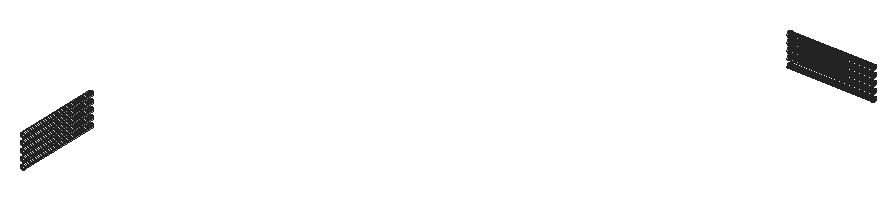
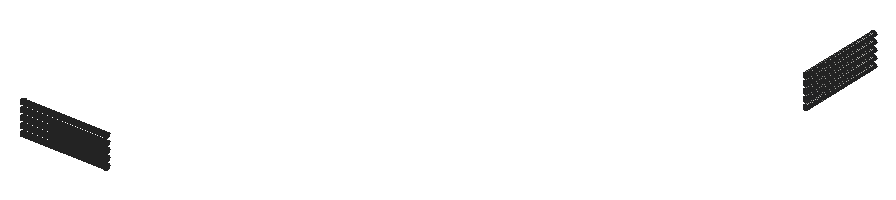
# SketchUp Ruby script. Lengths in inches.
U = 1.inch
M = Sketchup.active_model
def pt(a) = Geom::Point3d.new(a.map { |v| v * U })
def face(e, loops, mat)
  f = e.add_face(loops[0].map { |a| pt(a) })
  loops[1..].each { |l| e.add_face(l.map { |a| pt(a) }).erase! }
  f.material = f.back_material = mat if mat
  f
end
# faces: each face lists its corners as indices into pts; further lists are holes
def faces(e, pts, list, mat = nil) = list.each { |f| face(e, (f[0].is_a?(Array) ? f : [f]).map { |l| l.map { |i| pts[i] } }, mat) }
# xy, xz, yz: faces in a plane at the given z, y or x. An outline is a flat list of corners, or four numbers for a rectangle; further outlines are holes
def ring(l) = l.size == 4 ? [[l[0], l[1]], [l[2], l[1]], [l[2], l[3]], [l[0], l[3]]] : l.each_slice(2).to_a
def flat(e, list, mat, &to3) = list.each { |f| face(e, (f[0].is_a?(Array) ? f : [f]).map { |l| ring(l).map { |u, v| to3.(u, v) } }, mat) }
def xy(e, z, list, mat = nil) = flat(e, list, mat) { |x, y| [x, y, z] }
def xz(e, y, list, mat = nil) = flat(e, list, mat) { |x, z| [x, y, z] }
def yz(e, x, list, mat = nil) = flat(e, list, mat) { |y, z| [x, y, z] }
def lines(e, pts, list) = list.each { |a, b| e.add_line(pt(pts[a]), pt(pts[b])) }
# prism: a flat outline (further loops are holes) pulled along v
def prism(e, loops, v, mat = nil)
  f = face(e, loops, mat); d = Geom::Vector3d.new(v.map { |x| x * U })
  f.pushpull(f.normal.samedirection?(d) ? d.length : -d.length)
end
def box(e, o, s, mat = nil) = prism(e, [[o, [o[0] + s[0], o[1], o[2]], [o[0] + s[0], o[1] + s[1], o[2]], [o[0], o[1] + s[1], o[2]]]], [0, 0, s[2]], mat)
def at(x, y, z, deg = 0) = Geom::Transformation.translation(pt([x, y, z])) * Geom::Transformation.rotation(ORIGIN, Z_AXIS, deg.degrees)
def axes(o, x, y, z) = Geom::Transformation.new([*x, 0, *y, 0, *z, 0, *pt(o).to_a, 1])
def part(name) = M.definitions.add(name)
# library, detail: a bought-in or finely detailed component or shape, given as its bounding box
def library(name, o, s) = part(name).tap { |d| box(d.entities, o, s) }
def detail(e, o, s) = box(e.add_group.entities, o, s)
def put(e, d, t, mat = nil) = e.add_instance(d, t).tap { |i| i.material = mat if mat }
def group(e, t, mat = nil) = e.add_group.tap { |g| g.transformation = t; g.material = mat if mat }.entities
root = M.entities
p = [[83.53,662.8,1317.02],[82.57,662.8,1317.14],[82.57,806.17,1317.14],[83.53,806.17,1317.02],[84.48,662.8,1317.14],[84.48,806.17,1317.14],
  [697.99,1500.33,1317.14],[697.99,1501.28,1317.02],[841.36,1501.28,1317.02],[841.36,1500.33,1317.14],[697.99,1502.24,1317.14],[841.36,1502.24,1317.14],
  [81.68,662.8,1317.51],[81.68,806.17,1317.51],[85.37,662.8,1317.51],[85.37,806.17,1317.51],[697.99,1499.44,1317.51],[841.36,1499.44,1317.51],
  [697.99,1503.13,1317.51],[841.36,1503.13,1317.51],[80.92,662.8,1318.1],[80.92,806.17,1318.1],[86.13,662.8,1318.1],[86.13,806.17,1318.1],
  [697.99,1498.68,1318.1],[841.36,1498.68,1318.1],[697.99,1503.89,1318.1],[841.36,1503.89,1318.1],[80.33,662.8,1318.86],[80.33,806.17,1318.86],
  [86.72,662.8,1318.86],[86.72,806.17,1318.86],[697.99,1498.09,1318.86],[841.36,1498.09,1318.86],[697.99,1504.48,1318.86],[841.36,1504.48,1318.86],
  [79.97,662.8,1319.75],[79.97,806.17,1319.75],[87.09,662.8,1319.75],[87.09,806.17,1319.75],[697.99,1497.72,1319.75],[841.36,1497.72,1319.75],
  [697.99,1504.85,1319.75],[841.36,1504.85,1319.75],[79.84,662.8,1320.7],[79.84,806.17,1320.7],[87.21,662.8,1320.7],[87.21,806.17,1320.7],
  [697.99,1497.6,1320.7],[841.36,1497.6,1320.7],[697.99,1504.97,1320.7],[841.36,1504.97,1320.7],[79.97,662.8,1321.66],[79.97,806.17,1321.66],
  [87.09,662.8,1321.66],[87.09,806.17,1321.66],[697.99,1497.72,1321.66],[841.36,1497.72,1321.66],[697.99,1504.85,1321.66],[841.36,1504.85,1321.66],
  [80.33,662.8,1322.55],[80.33,806.17,1322.55],[86.72,662.8,1322.55],[86.72,806.17,1322.55],[697.99,1498.09,1322.55],[841.36,1498.09,1322.55],
  [697.99,1504.48,1322.55],[841.36,1504.48,1322.55],[80.92,662.8,1323.3125],[80.92,806.17,1323.3125],[86.13,662.8,1323.3125],[86.13,806.17,1323.3125],
  [697.99,1498.68,1323.3125],[841.36,1498.68,1323.3125],[697.99,1503.89,1323.3125],[841.36,1503.89,1323.3125],[81.68,662.8,1323.9],[81.68,806.17,1323.9],
  [85.37,662.8,1323.9],[85.37,806.17,1323.9],[697.99,1499.44,1323.9],[841.36,1499.44,1323.9],[697.99,1503.13,1323.9],[841.36,1503.13,1323.9],
  [82.57,662.8,1324.27],[82.57,806.17,1324.27],[84.48,662.8,1324.27],[84.48,806.17,1324.27],[697.99,1500.33,1324.27],[841.36,1500.33,1324.27],
  [697.99,1502.24,1324.27],[841.36,1502.24,1324.27],[83.53,662.8,1324.39],[83.53,806.17,1324.39],[697.99,1501.28,1324.39],[841.36,1501.28,1324.39],
  [83.53,662.8,1329.02],[82.57,662.8,1329.14],[82.57,806.17,1329.14],[83.53,806.17,1329.02],[84.48,662.8,1329.14],[84.48,806.17,1329.14],
  [697.99,1500.33,1329.14],[697.99,1501.28,1329.02],[841.36,1501.28,1329.02],[841.36,1500.33,1329.14],[697.99,1502.24,1329.14],[841.36,1502.24,1329.14],
  [81.68,662.8,1329.51],[81.68,806.17,1329.51],[85.37,662.8,1329.51],[85.37,806.17,1329.51],[697.99,1499.44,1329.51],[841.36,1499.44,1329.51],
  [697.99,1503.13,1329.51],[841.36,1503.13,1329.51],[80.92,662.8,1330.1],[80.92,806.17,1330.1],[86.13,662.8,1330.1],[86.13,806.17,1330.1],
  [697.99,1498.68,1330.1],[841.36,1498.68,1330.1],[697.99,1503.89,1330.1],[841.36,1503.89,1330.1],[80.33,662.8,1330.86],[80.33,806.17,1330.86],
  [86.72,662.8,1330.86],[86.72,806.17,1330.86],[697.99,1498.09,1330.86],[841.36,1498.09,1330.86],[697.99,1504.48,1330.86],[841.36,1504.48,1330.86],
  [79.97,662.8,1331.75],[79.97,806.17,1331.75],[87.09,662.8,1331.75],[87.09,806.17,1331.75],[697.99,1497.72,1331.75],[841.36,1497.72,1331.75],
  [697.99,1504.85,1331.75],[841.36,1504.85,1331.75],[79.84,662.8,1332.7],[79.84,806.17,1332.7],[87.21,662.8,1332.7],[87.21,806.17,1332.7],
  [697.99,1497.6,1332.7],[841.36,1497.6,1332.7],[697.99,1504.97,1332.7],[841.36,1504.97,1332.7],[79.97,662.8,1333.66],[79.97,806.17,1333.66],
  [87.09,662.8,1333.66],[87.09,806.17,1333.66],[697.99,1497.72,1333.66],[841.36,1497.72,1333.66],[697.99,1504.85,1333.66],[841.36,1504.85,1333.66],
  [80.33,662.8,1334.55],[80.33,806.17,1334.55],[86.72,662.8,1334.55],[86.72,806.17,1334.55],[697.99,1498.09,1334.55],[841.36,1498.09,1334.55],
  [697.99,1504.48,1334.55],[841.36,1504.48,1334.55],[80.92,662.8,1335.3125],[80.92,806.17,1335.3125],[86.13,662.8,1335.3125],[86.13,806.17,1335.3125],
  [697.99,1498.68,1335.3125],[841.36,1498.68,1335.3125],[697.99,1503.89,1335.3125],[841.36,1503.89,1335.3125],[81.68,662.8,1335.9],[81.68,806.17,1335.9],
  [85.37,662.8,1335.9],[85.37,806.17,1335.9],[697.99,1499.44,1335.9],[841.36,1499.44,1335.9],[697.99,1503.13,1335.9],[841.36,1503.13,1335.9],
  [82.57,662.8,1336.27],[82.57,806.17,1336.27],[84.48,662.8,1336.27],[84.48,806.17,1336.27],[697.99,1500.33,1336.27],[841.36,1500.33,1336.27],
  [697.99,1502.24,1336.27],[841.36,1502.24,1336.27],[83.53,662.8,1336.39],[83.53,806.17,1336.39],[697.99,1501.28,1336.39],[841.36,1501.28,1336.39],
  [83.53,662.8,1341.02],[82.57,662.8,1341.14],[82.57,806.17,1341.14],[83.53,806.17,1341.02],[84.48,662.8,1341.14],[84.48,806.17,1341.14],
  [697.99,1500.33,1341.14],[697.99,1501.28,1341.02],[841.36,1501.28,1341.02],[841.36,1500.33,1341.14],[697.99,1502.24,1341.14],[841.36,1502.24,1341.14],
  [81.68,662.8,1341.51],[81.68,806.17,1341.51],[85.37,662.8,1341.51],[85.37,806.17,1341.51],[697.99,1499.44,1341.51],[841.36,1499.44,1341.51],
  [697.99,1503.13,1341.51],[841.36,1503.13,1341.51],[80.92,662.8,1342.1],[80.92,806.17,1342.1],[86.13,662.8,1342.1],[86.13,806.17,1342.1],
  [697.99,1498.68,1342.1],[841.36,1498.68,1342.1],[697.99,1503.89,1342.1],[841.36,1503.89,1342.1],[80.33,662.8,1342.86],[80.33,806.17,1342.86],
  [86.72,662.8,1342.86],[86.72,806.17,1342.86],[697.99,1498.09,1342.86],[841.36,1498.09,1342.86],[697.99,1504.48,1342.86],[841.36,1504.48,1342.86],
  [79.97,662.8,1343.75],[79.97,806.17,1343.75],[87.09,662.8,1343.75],[87.09,806.17,1343.75],[697.99,1497.72,1343.75],[841.36,1497.72,1343.75],
  [697.99,1504.85,1343.75],[841.36,1504.85,1343.75],[79.84,662.8,1344.7],[79.84,806.17,1344.7],[87.21,662.8,1344.7],[87.21,806.17,1344.7],
  [697.99,1497.6,1344.7],[841.36,1497.6,1344.7],[697.99,1504.97,1344.7],[841.36,1504.97,1344.7],[79.97,662.8,1345.66],[79.97,806.17,1345.66],
  [87.09,662.8,1345.66],[87.09,806.17,1345.66],[697.99,1497.72,1345.66],[841.36,1497.72,1345.66],[697.99,1504.85,1345.66],[841.36,1504.85,1345.66],
  [80.33,662.8,1346.55],[80.33,806.17,1346.55],[86.72,662.8,1346.55],[86.72,806.17,1346.55],[697.99,1498.09,1346.55],[841.36,1498.09,1346.55],
  [697.99,1504.48,1346.55],[841.36,1504.48,1346.55],[80.92,662.8,1347.3125],[80.92,806.17,1347.3125],[86.13,662.8,1347.3125],[86.13,806.17,1347.3125],
  [697.99,1498.68,1347.3125],[841.36,1498.68,1347.3125],[697.99,1503.89,1347.3125],[841.36,1503.89,1347.3125],[81.68,662.8,1347.9],[81.68,806.17,1347.9],
  [85.37,662.8,1347.9],[85.37,806.17,1347.9],[697.99,1499.44,1347.9],[841.36,1499.44,1347.9],[697.99,1503.13,1347.9],[841.36,1503.13,1347.9],
  [82.57,662.8,1348.27],[82.57,806.17,1348.27],[84.48,662.8,1348.27],[84.48,806.17,1348.27],[697.99,1500.33,1348.27],[841.36,1500.33,1348.27],
  [697.99,1502.24,1348.27],[841.36,1502.24,1348.27],[83.53,662.8,1348.39],[83.53,806.17,1348.39],[697.99,1501.28,1348.39],[841.36,1501.28,1348.39],
  [83.53,662.8,1353.02],[82.57,662.8,1353.14],[82.57,806.17,1353.14],[83.53,806.17,1353.02],[84.48,662.8,1353.14],[84.48,806.17,1353.14],
  [697.99,1500.33,1353.14],[697.99,1501.28,1353.02],[841.36,1501.28,1353.02],[841.36,1500.33,1353.14],[697.99,1502.24,1353.14],[841.36,1502.24,1353.14],
  [81.68,662.8,1353.51],[81.68,806.17,1353.51],[85.37,662.8,1353.51],[85.37,806.17,1353.51],[697.99,1499.44,1353.51],[841.36,1499.44,1353.51],
  [697.99,1503.13,1353.51],[841.36,1503.13,1353.51],[80.92,662.8,1354.1],[80.92,806.17,1354.1],[86.13,662.8,1354.1],[86.13,806.17,1354.1],
  [697.99,1498.68,1354.1],[841.36,1498.68,1354.1],[697.99,1503.89,1354.1],[841.36,1503.89,1354.1],[80.33,662.8,1354.86],[80.33,806.17,1354.86],
  [86.72,662.8,1354.86],[86.72,806.17,1354.86],[697.99,1498.09,1354.86],[841.36,1498.09,1354.86],[697.99,1504.48,1354.86],[841.36,1504.48,1354.86],
  [79.97,662.8,1355.75],[79.97,806.17,1355.75],[87.09,662.8,1355.75],[87.09,806.17,1355.75],[697.99,1497.72,1355.75],[841.36,1497.72,1355.75],
  [697.99,1504.85,1355.75],[841.36,1504.85,1355.75],[79.84,662.8,1356.7],[79.84,806.17,1356.7],[87.21,662.8,1356.7],[87.21,806.17,1356.7],
  [697.99,1497.6,1356.7],[841.36,1497.6,1356.7],[697.99,1504.97,1356.7],[841.36,1504.97,1356.7],[79.97,662.8,1357.66],[79.97,806.17,1357.66],
  [87.09,662.8,1357.66],[87.09,806.17,1357.66],[697.99,1497.72,1357.66],[841.36,1497.72,1357.66],[697.99,1504.85,1357.66],[841.36,1504.85,1357.66],
  [80.33,662.8,1358.55],[80.33,806.17,1358.55],[86.72,662.8,1358.55],[86.72,806.17,1358.55],[697.99,1498.09,1358.55],[841.36,1498.09,1358.55],
  [697.99,1504.48,1358.55],[841.36,1504.48,1358.55],[80.92,662.8,1359.3125],[80.92,806.17,1359.3125],[86.13,662.8,1359.3125],[86.13,806.17,1359.3125],
  [697.99,1498.68,1359.3125],[841.36,1498.68,1359.3125],[697.99,1503.89,1359.3125],[841.36,1503.89,1359.3125],[81.68,662.8,1359.9],[81.68,806.17,1359.9],
  [85.37,662.8,1359.9],[85.37,806.17,1359.9],[697.99,1499.44,1359.9],[841.36,1499.44,1359.9],[697.99,1503.13,1359.9],[841.36,1503.13,1359.9],
  [82.57,662.8,1360.27],[82.57,806.17,1360.27],[84.48,662.8,1360.27],[84.48,806.17,1360.27],[697.99,1500.33,1360.27],[841.36,1500.33,1360.27],
  [697.99,1502.24,1360.27],[841.36,1502.24,1360.27],[83.53,662.8,1360.39],[83.53,806.17,1360.39],[697.99,1501.28,1360.39],[841.36,1501.28,1360.39],
  [83.53,662.8,1365.02],[82.57,662.8,1365.14],[82.57,806.17,1365.14],[83.53,806.17,1365.02],[84.48,662.8,1365.14],[84.48,806.17,1365.14],
  [697.99,1500.33,1365.14],[697.99,1501.28,1365.02],[841.36,1501.28,1365.02],[841.36,1500.33,1365.14],[697.99,1502.24,1365.14],[841.36,1502.24,1365.14],
  [81.68,662.8,1365.51],[81.68,806.17,1365.51],[85.37,662.8,1365.51],[85.37,806.17,1365.51],[697.99,1499.44,1365.51],[841.36,1499.44,1365.51],
  [697.99,1503.13,1365.51],[841.36,1503.13,1365.51],[80.92,662.8,1366.1],[80.92,806.17,1366.1],[86.13,662.8,1366.1],[86.13,806.17,1366.1],
  [697.99,1498.68,1366.1],[841.36,1498.68,1366.1],[697.99,1503.89,1366.1],[841.36,1503.89,1366.1],[80.33,662.8,1366.86],[80.33,806.17,1366.86],
  [86.72,662.8,1366.86],[86.72,806.17,1366.86],[697.99,1498.09,1366.86],[841.36,1498.09,1366.86],[697.99,1504.48,1366.86],[841.36,1504.48,1366.86],
  [79.97,662.8,1367.75],[79.97,806.17,1367.75],[87.09,662.8,1367.75],[87.09,806.17,1367.75],[697.99,1497.72,1367.75],[841.36,1497.72,1367.75],
  [697.99,1504.85,1367.75],[841.36,1504.85,1367.75],[79.84,662.8,1368.7],[79.84,806.17,1368.7],[87.21,662.8,1368.7],[87.21,806.17,1368.7],
  [697.99,1497.6,1368.7],[841.36,1497.6,1368.7],[697.99,1504.97,1368.7],[841.36,1504.97,1368.7],[79.97,662.8,1369.66],[79.97,806.17,1369.66],
  [87.09,662.8,1369.66],[87.09,806.17,1369.66],[697.99,1497.72,1369.66],[841.36,1497.72,1369.66],[697.99,1504.85,1369.66],[841.36,1504.85,1369.66],
  [80.33,662.8,1370.55],[80.33,806.17,1370.55],[86.72,662.8,1370.55],[86.72,806.17,1370.55],[697.99,1498.09,1370.55],[841.36,1498.09,1370.55],
  [697.99,1504.48,1370.55],[841.36,1504.48,1370.55],[80.92,662.8,1371.3125],[80.92,806.17,1371.3125],[86.13,662.8,1371.3125],[86.13,806.17,1371.3125],
  [697.99,1498.68,1371.3125],[841.36,1498.68,1371.3125],[697.99,1503.89,1371.3125],[841.36,1503.89,1371.3125],[81.68,662.8,1371.9],[81.68,806.17,1371.9],
  [85.37,662.8,1371.9],[85.37,806.17,1371.9],[697.99,1499.44,1371.9],[841.36,1499.44,1371.9],[697.99,1503.13,1371.9],[841.36,1503.13,1371.9],
  [82.57,662.8,1372.27],[82.57,806.17,1372.27],[84.48,662.8,1372.27],[84.48,806.17,1372.27],[697.99,1500.33,1372.27],[841.36,1500.33,1372.27],
  [697.99,1502.24,1372.27],[841.36,1502.24,1372.27],[83.53,662.8,1372.39],[83.53,806.17,1372.39],[697.99,1501.28,1372.39],[841.36,1501.28,1372.39]]
faces(root,p,[[0,1,2,3],[4,0,3,5],[6,7,8,9],[7,10,11,8],[1,12,13,2],[14,4,5,15],[16,6,9,17],[10,18,19,11],
  [12,20,21,13],[22,14,15,23],[24,16,17,25],[18,26,27,19],[20,28,29,21],[30,22,23,31],[32,24,25,33],[26,34,35,27],
  [28,36,37,29],[38,30,31,39],[40,32,33,41],[34,42,43,35],[36,44,45,37],[46,38,39,47],[48,40,41,49],[42,50,51,43],
  [44,52,53,45],[54,46,47,55],[56,48,49,57],[50,58,59,51],[52,60,61,53],[62,54,55,63],[64,56,57,65],[58,66,67,59],
  [60,68,69,61],[70,62,63,71],[72,64,65,73],[66,74,75,67],[68,76,77,69],[78,70,71,79],[80,72,73,81],[74,82,83,75],
  [76,84,85,77],[86,78,79,87],[88,80,81,89],[82,90,91,83],[84,92,93,85],[92,86,87,93],[94,88,89,95],[90,94,95,91],
  [96,97,98,99],[100,96,99,101],[102,103,104,105],[103,106,107,104],[97,108,109,98],[110,100,101,111],[112,102,105,113],[106,114,115,107],
  [108,116,117,109],[118,110,111,119],[120,112,113,121],[114,122,123,115],[116,124,125,117],[126,118,119,127],[128,120,121,129],[122,130,131,123],
  [124,132,133,125],[134,126,127,135],[136,128,129,137],[130,138,139,131],[132,140,141,133],[142,134,135,143],[144,136,137,145],[138,146,147,139],
  [140,148,149,141],[150,142,143,151],[152,144,145,153],[146,154,155,147],[148,156,157,149],[158,150,151,159],[160,152,153,161],[154,162,163,155],
  [156,164,165,157],[166,158,159,167],[168,160,161,169],[162,170,171,163],[164,172,173,165],[174,166,167,175],[176,168,169,177],[170,178,179,171],
  [172,180,181,173],[182,174,175,183],[184,176,177,185],[178,186,187,179],[180,188,189,181],[188,182,183,189],[190,184,185,191],[186,190,191,187],
  [192,193,194,195],[196,192,195,197],[198,199,200,201],[199,202,203,200],[193,204,205,194],[206,196,197,207],[208,198,201,209],[202,210,211,203],
  [204,212,213,205],[214,206,207,215],[216,208,209,217],[210,218,219,211],[212,220,221,213],[222,214,215,223],[224,216,217,225],[218,226,227,219],
  [220,228,229,221],[230,222,223,231],[232,224,225,233],[226,234,235,227],[228,236,237,229],[238,230,231,239],[240,232,233,241],[234,242,243,235],
  [236,244,245,237],[246,238,239,247],[248,240,241,249],[242,250,251,243],[244,252,253,245],[254,246,247,255],[256,248,249,257],[250,258,259,251],
  [252,260,261,253],[262,254,255,263],[264,256,257,265],[258,266,267,259],[260,268,269,261],[270,262,263,271],[272,264,265,273],[266,274,275,267],
  [268,276,277,269],[278,270,271,279],[280,272,273,281],[274,282,283,275],[276,284,285,277],[284,278,279,285],[286,280,281,287],[282,286,287,283],
  [288,289,290,291],[292,288,291,293],[294,295,296,297],[295,298,299,296],[289,300,301,290],[302,292,293,303],[304,294,297,305],[298,306,307,299],
  [300,308,309,301],[310,302,303,311],[312,304,305,313],[306,314,315,307],[308,316,317,309],[318,310,311,319],[320,312,313,321],[314,322,323,315],
  [316,324,325,317],[326,318,319,327],[328,320,321,329],[322,330,331,323],[324,332,333,325],[334,326,327,335],[336,328,329,337],[330,338,339,331],
  [332,340,341,333],[342,334,335,343],[344,336,337,345],[338,346,347,339],[340,348,349,341],[350,342,343,351],[352,344,345,353],[346,354,355,347],
  [348,356,357,349],[358,350,351,359],[360,352,353,361],[354,362,363,355],[356,364,365,357],[366,358,359,367],[368,360,361,369],[362,370,371,363],
  [364,372,373,365],[374,366,367,375],[376,368,369,377],[370,378,379,371],[372,380,381,373],[380,374,375,381],[382,376,377,383],[378,382,383,379],
  [384,385,386,387],[388,384,387,389],[390,391,392,393],[391,394,395,392],[385,396,397,386],[398,388,389,399],[400,390,393,401],[394,402,403,395],
  [396,404,405,397],[406,398,399,407],[408,400,401,409],[402,410,411,403],[404,412,413,405],[414,406,407,415],[416,408,409,417],[410,418,419,411],
  [412,420,421,413],[422,414,415,423],[424,416,417,425],[418,426,427,419],[420,428,429,421],[430,422,423,431],[432,424,425,433],[426,434,435,427],
  [428,436,437,429],[438,430,431,439],[440,432,433,441],[434,442,443,435],[436,444,445,437],[446,438,439,447],[448,440,441,449],[442,450,451,443],
  [444,452,453,445],[454,446,447,455],[456,448,449,457],[450,458,459,451],[452,460,461,453],[462,454,455,463],[464,456,457,465],[458,466,467,459],
  [460,468,469,461],[470,462,463,471],[472,464,465,473],[466,474,475,467],[468,476,477,469],[476,470,471,477],[478,472,473,479],[474,478,479,475]])
